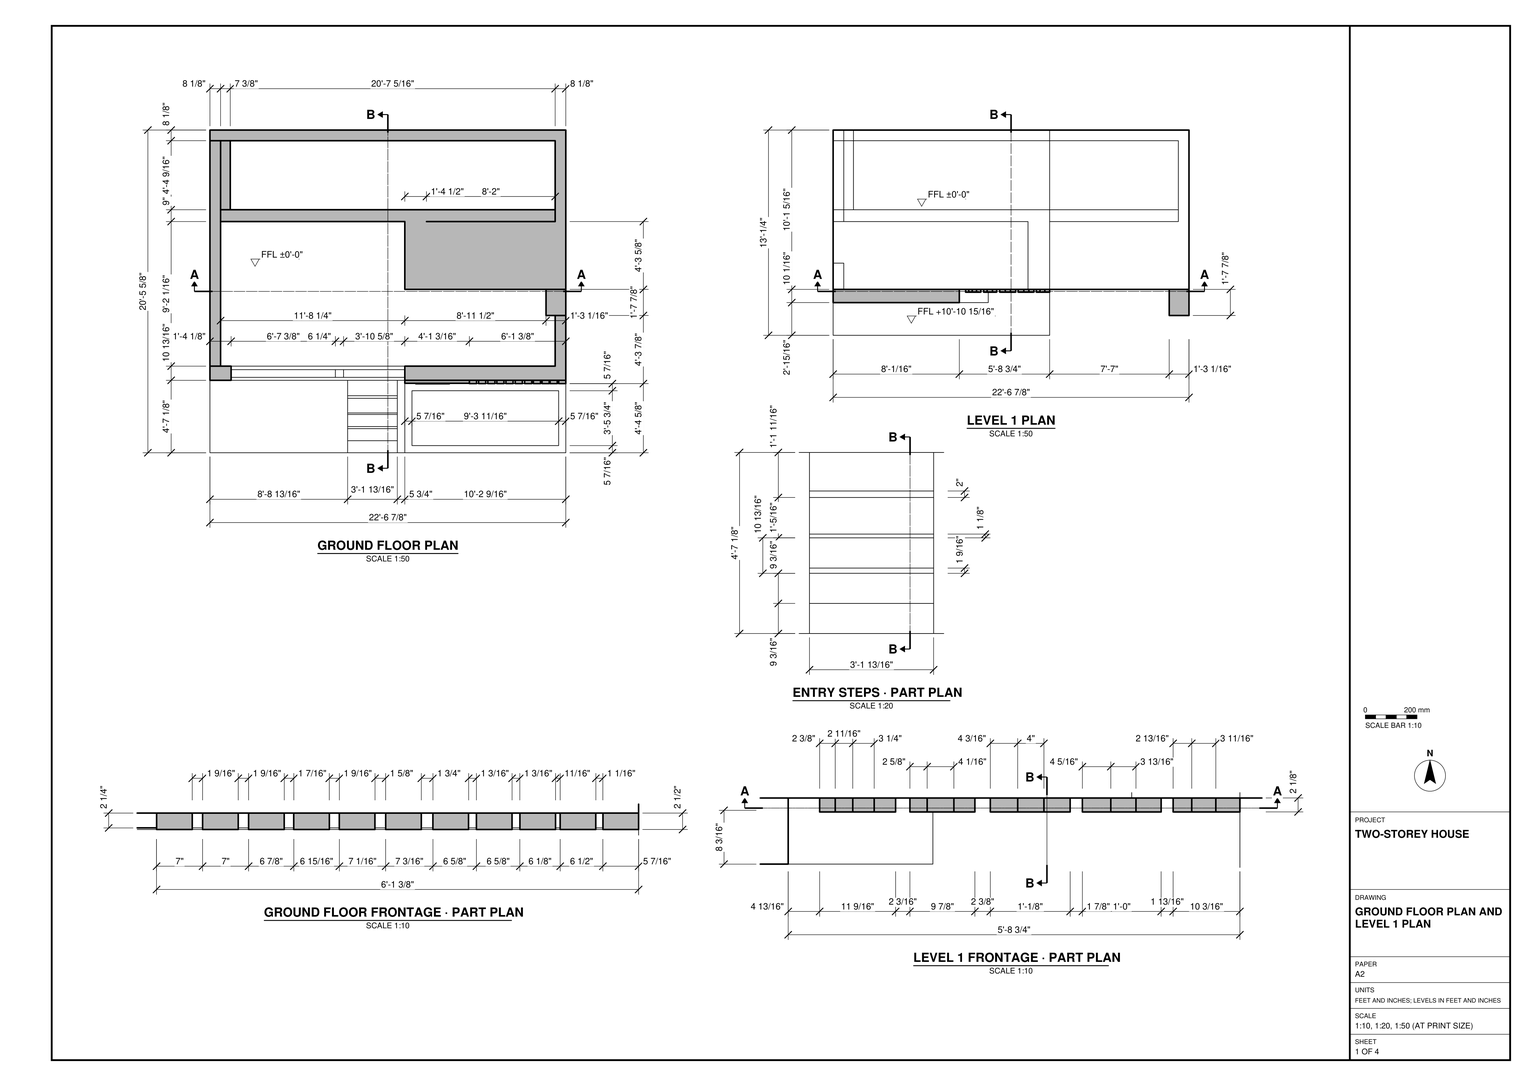
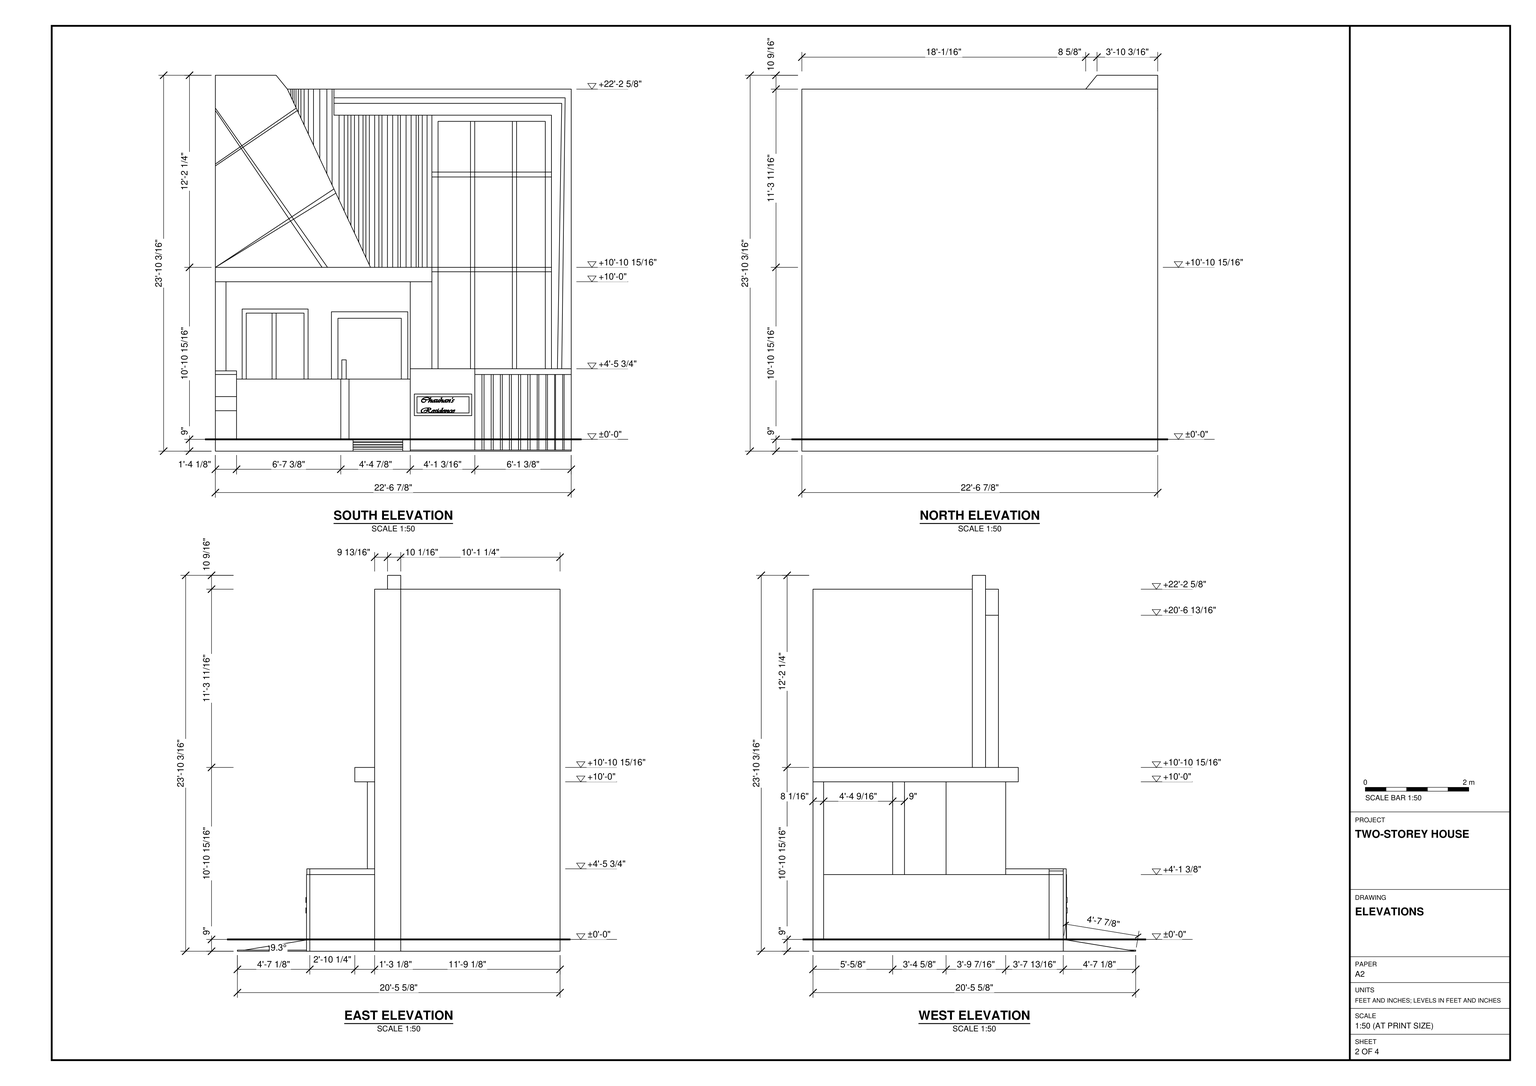
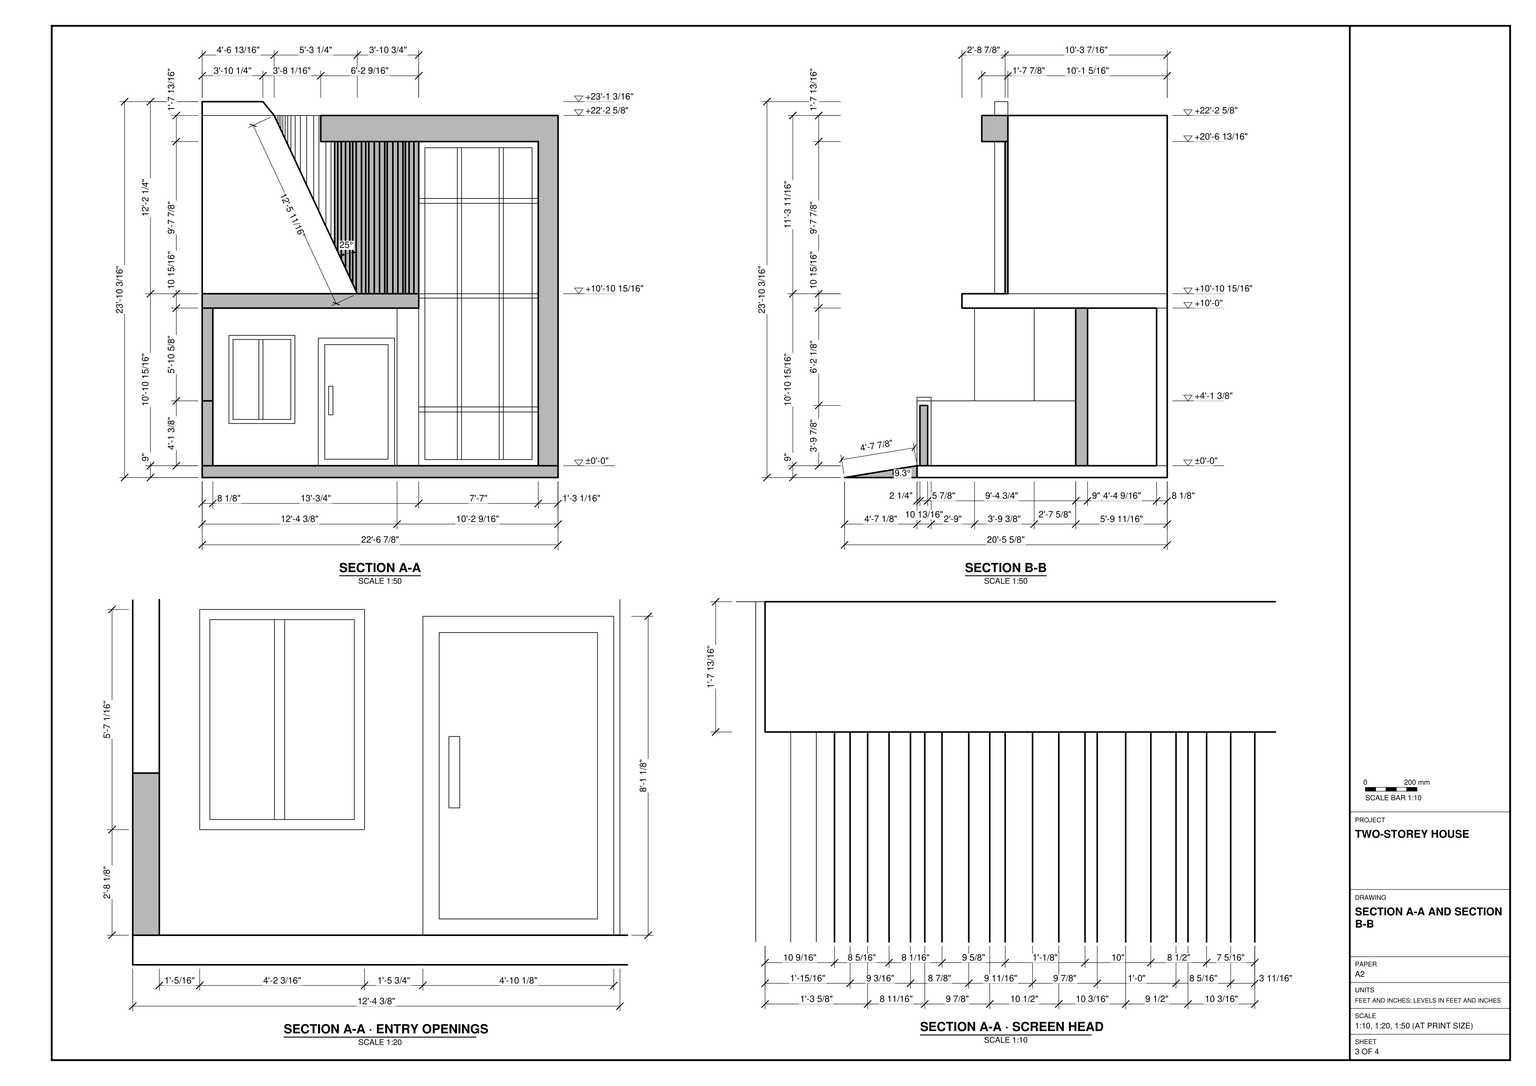
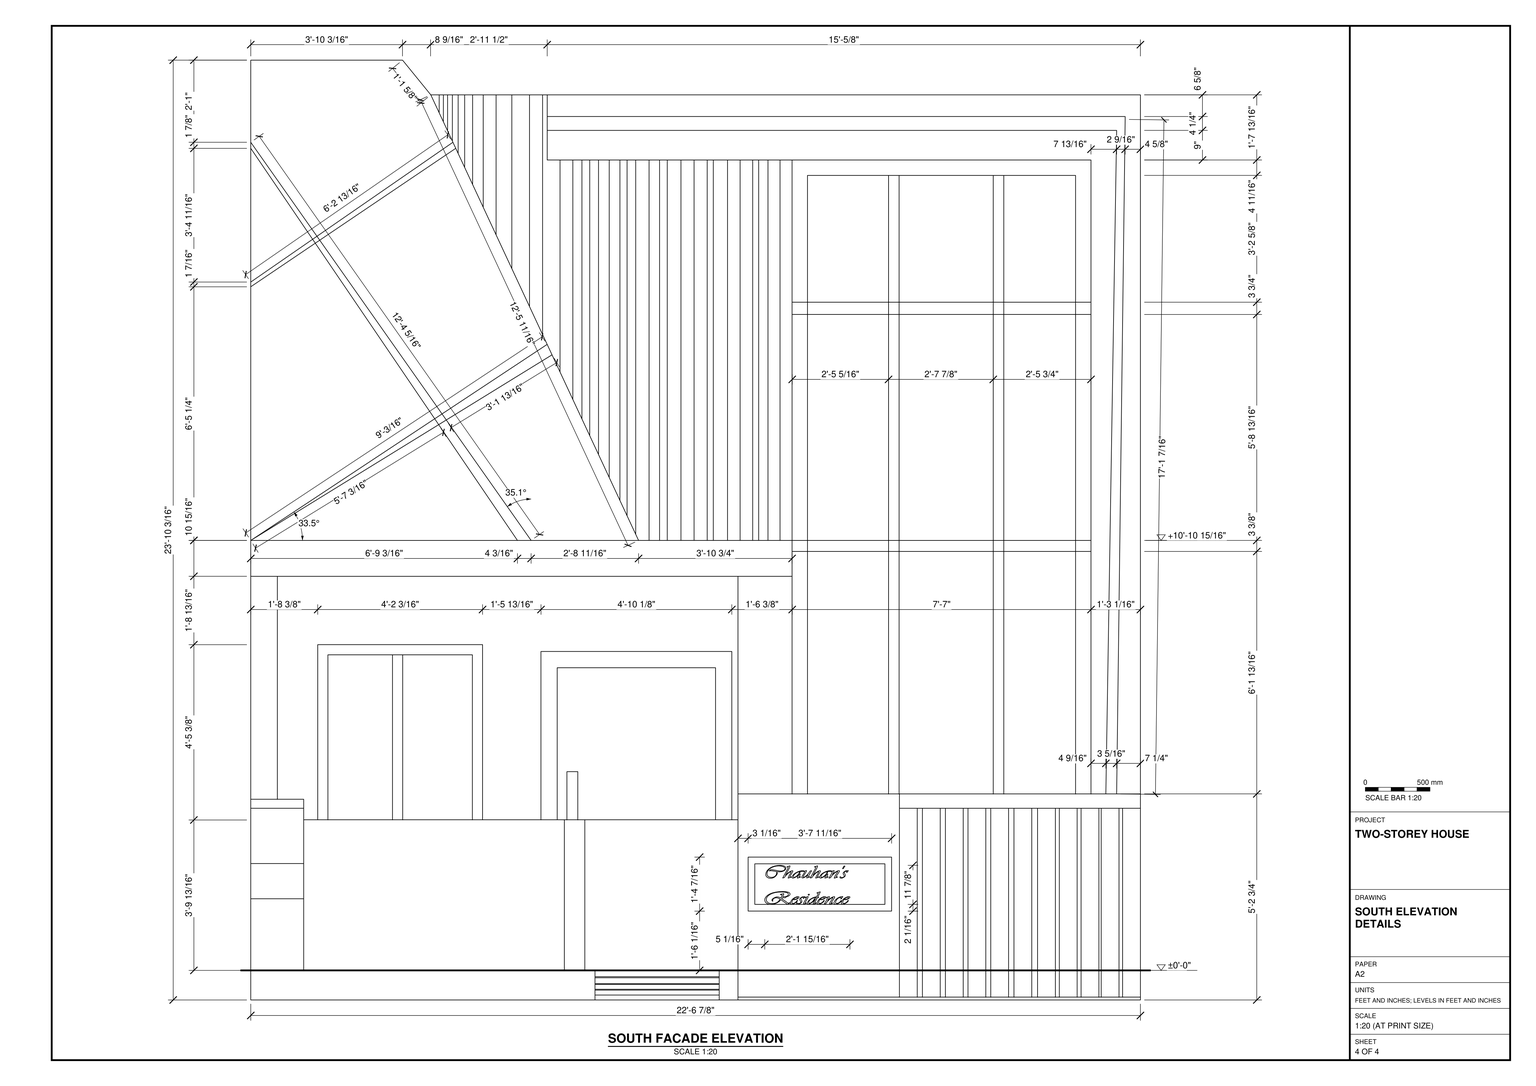
Build the two-storey house in SketchUp from task_files/diagram_01.pdf. Work in feet and inches. The overall dimensions are 22'-6 7/8" across the south frontage, 20'-5 5/8" from front to back and 23'-10 3/16" high. Set the ground floor at ±0'-0" and Level 1 at +10'-10 15/16".

Use the plans to set out the walls at their drawn thicknesses and the sections to locate the base slab, projecting Level 1 slab and roof edge. At the south entrance, model the steps, adjoining sloped approach and low frontage elements. Set the framed door and divided window back from the frontage, beneath the projecting slab. To their right, carry the tall glazed bay past Level 1 without interrupting it with the slab edge. Match its mullions, horizontal divisions and outer frame to section A-A. Above the entrance, fit the vertical screen between the glazed bay and the panel with the sloping edge. Follow the south elevation for the diagonal joints on that panel and the part plans for the spacing of the frontage members.

Keep walls, slabs and roof elements in separate groups or components. Group each furniture or joinery piece separately and use components for repeated parts. Any decor or loose items shown may be represented by suitable library components. Save one SketchUp model as output_files/two_storey_house_with_a_screened_south_frontage.skp.

# SketchUp Ruby script. Lengths in inches.
U = 1.inch
M = Sketchup.active_model
def pt(a) = Geom::Point3d.new(a.map { |v| v * U })
def face(e, loops, mat)
  f = e.add_face(loops[0].map { |a| pt(a) })
  loops[1..].each { |l| e.add_face(l.map { |a| pt(a) }).erase! }
  f.material = f.back_material = mat if mat
  f
end
# faces: each face lists its corners as indices into pts; further lists are holes
def faces(e, pts, list, mat = nil) = list.each { |f| face(e, (f[0].is_a?(Array) ? f : [f]).map { |l| l.map { |i| pts[i] } }, mat) }
# xy, xz, yz: faces in a plane at the given z, y or x. An outline is a flat list of corners, or four numbers for a rectangle; further outlines are holes
def ring(l) = l.size == 4 ? [[l[0], l[1]], [l[2], l[1]], [l[2], l[3]], [l[0], l[3]]] : l.each_slice(2).to_a
def flat(e, list, mat, &to3) = list.each { |f| face(e, (f[0].is_a?(Array) ? f : [f]).map { |l| ring(l).map { |u, v| to3.(u, v) } }, mat) }
def xy(e, z, list, mat = nil) = flat(e, list, mat) { |x, y| [x, y, z] }
def xz(e, y, list, mat = nil) = flat(e, list, mat) { |x, z| [x, y, z] }
def yz(e, x, list, mat = nil) = flat(e, list, mat) { |y, z| [x, y, z] }
def lines(e, pts, list) = list.each { |a, b| e.add_line(pt(pts[a]), pt(pts[b])) }
# prism: a flat outline (further loops are holes) pulled along v
def prism(e, loops, v, mat = nil)
  f = face(e, loops, mat); d = Geom::Vector3d.new(v.map { |x| x * U })
  f.pushpull(f.normal.samedirection?(d) ? d.length : -d.length)
end
def box(e, o, s, mat = nil) = prism(e, [[o, [o[0] + s[0], o[1], o[2]], [o[0] + s[0], o[1] + s[1], o[2]], [o[0], o[1] + s[1], o[2]]]], [0, 0, s[2]], mat)
def at(x, y, z, deg = 0) = Geom::Transformation.translation(pt([x, y, z])) * Geom::Transformation.rotation(ORIGIN, Z_AXIS, deg.degrees)
def axes(o, x, y, z) = Geom::Transformation.new([*x, 0, *y, 0, *z, 0, *pt(o).to_a, 1])
def part(name) = M.definitions.add(name)
# library, detail: a bought-in or finely detailed component or shape, given as its bounding box
def library(name, o, s) = part(name).tap { |d| box(d.entities, o, s) }
def detail(e, o, s) = box(e.add_group.entities, o, s)
def put(e, d, t, mat = nil) = e.add_instance(d, t).tap { |i| i.material = mat if mat }
def group(e, t, mat = nil) = e.add_group.tap { |g| g.transformation = t; g.material = mat if mat }.entities
root = M.entities
M.materials.add("[0014_DarkSalmon]").color = [242, 155, 126]
M.materials.add("[Asphalt New]").color = [67, 60, 62]
M.materials.add("[Blacktop New]").color = [81, 81, 81]
M.materials.add("[Concrete Aggregate Smoke]").color = [154, 150, 148]
M.materials.add("[Concrete Form 4x8]").color = [167, 170, 168]
M.materials.add("[Formica Beige]").color = [211, 187, 149]
M.materials.add("[Formica Graystone]").color = [149, 146, 135]
M.materials.add("[Formica Laminate Dark]").color = [50, 53, 60]
M.materials.add("[Formica Laminate Light]").color = [213, 189, 164]
M.materials.add("[Formica Speckled Grey]").color = [94, 105, 111]
M.materials.add("[Grass Dark Green]").color = [106, 157, 55]
M.materials.add("[Marble Carrara Floor Tile]").color = [204, 208, 219]
M.materials.add("[Marble Carrara Gold Floor Tile]").color = [225, 223, 217]
M.materials.add("[Polished Concrete New]").color = [200, 200, 203]
M.materials.add("[Polished Concrete Old]").color = [229, 229, 229]
M.materials.add("[Terrazzo Tile Accent]").color = [224, 221, 217]
M.materials.add("[Translucent Glass Safety]").color = [204, 235, 244]
M.materials["[Translucent Glass Safety]"].alpha = 0.5
M.materials.add("[Translucent Resin Crush Gray]").color = [184, 184, 184]
M.materials["[Translucent Resin Crush Gray]"].alpha = 0.8
M.materials.add("[Wood Cherry Original]").color = [119, 67, 33]
M.materials.add("[Wood Cherry Original]1").color = [152, 86, 42]
M.materials.add("[Wood Veneer 01]").color = [76, 44, 23]
c1 = library("Chauhan's Reside",[0.93,0,0],[38.14,23.39,12])
xy(root,0,[[0,0,148.36,55.13],[[148.36,0,270.9,52.63],[153.79,5.43,265.47,47.2]],[148.36,52.63,197.52,52.88],[197.52,52.63,202.95,52.88],[202.95,52.63,204.52,52.88],
  [204.52,52.63,209.95,52.88],[209.95,52.63,211.52,52.88],[211.52,52.63,216.95,52.88],[216.95,52.63,218.4,52.88],[218.4,52.63,223.82,52.88],
  [223.82,52.63,225.33,52.88],[225.33,52.63,230.76,52.88],[230.76,52.63,232.4,52.88],[232.4,52.63,237.82,52.88],[237.82,52.63,239.58,52.88],
  [239.58,52.63,245.01,52.88],[245.01,52.63,246.21,52.88],[246.21,52.63,251.63,52.88],[251.63,52.63,252.83,52.88],[252.83,52.63,258.26,52.88],
  [258.26,52.63,258.96,52.88],[258.96,52.63,264.38,52.88],[264.38,52.63,265.48,52.88],[265.48,52.63,270.9,52.88],[148.36,52.88,197.52,55.13],
  [197.52,52.88,202.95,55.13],[202.95,52.88,204.52,55.13],[204.52,52.88,209.95,55.13],[209.95,52.88,211.52,55.13],[211.52,52.88,216.95,55.13],
  [216.95,52.88,218.4,55.13],[218.4,52.88,223.82,55.13],[223.82,52.88,225.33,55.13],[225.33,52.88,230.76,55.13],[230.76,52.88,232.4,55.13],
  [232.4,52.88,237.82,55.13],[237.82,52.88,239.58,55.13],[239.58,52.88,245.01,55.13],[245.01,52.88,246.21,55.13],[246.21,52.88,251.63,55.13],
  [251.63,52.88,252.83,55.13],[252.83,52.88,258.26,55.13],[258.26,52.88,258.96,55.13],[258.96,52.88,264.38,55.13],[264.38,52.88,265.48,55.13],
  [265.48,52.88,270.9,55.13],[0,55.13,270.9,245.65]])
xy(root,0,[[153.79,5.43,265.47,47.2]],"[Grass Dark Green]")
xy(root,0.875,[[[148.36,0,270.9,52.63],[153.79,5.43,265.47,47.2]]],"[Translucent Resin Crush Gray]")
xy(root,9,[[16.12,55.13,148.36,57.38],[16.12,57.38,148.36,63.26],[16.12,63.26,148.36,65.92],[0,65.92,8.1,237.55],[255.85,104.48,262.81,124.36],
  [262.81,104.48,270.9,124.36],[148.36,124.36,164.83,175.99],[8.1,175.99,262.81,185],[8.1,185,15.48,237.55],[15.48,185,262.81,237.55]])
xy(root,9,[[8.1,65.92,262.81,65.92,262.81,104.48,255.85,104.48,255.85,124.36,148.36,124.36,148.36,175.99,8.1,175.99]],"[Marble Carrara Floor Tile]")
xy(root,54.875,[[95.49,57.38,101.72,63.26]],"[Formica Graystone]")
xy(root,54.875,[[16.12,57.38,95.49,63.26],[101.72,57.38,148.36,63.26]],"[Formica Laminate Dark]")
xy(root,58.375,[[0,55.13,16.12,65.92],[148.36,55.13,148.36,65.92,262.81,65.92,262.81,104.48,270.9,104.48,270.9,55.13],[0,98.95,8.1,144.35]])
xy(root,58.375,[[0,65.92,8.1,98.95],[0,144.35,8.1,237.55]],"[Formica Graystone]")
xy(root,58.375,[[197.52,52.63,202.95,55.13],[204.52,52.63,209.95,55.13],[211.52,52.63,216.95,55.13],[218.4,52.63,223.82,55.13],[225.33,52.63,230.76,55.13],
  [232.4,52.63,237.82,55.13],[239.58,52.63,245.01,55.13],[246.21,52.63,251.63,55.13],[252.83,52.63,258.26,55.13],[258.96,52.63,264.38,55.13],
  [265.48,52.63,270.9,55.13]],"[Wood Cherry Original]1")
xy(root,61.125,[[0,55.13,16.12,65.92]],"[Asphalt New]")
xy(root,62.75,[[148.36,52.88,197.52,55.13]])
xy(root,62.75,[[148.36,55.13,270.9,55.13,270.9,104.48,262.81,104.48,262.81,65.92,148.36,65.92]],"[Asphalt New]")
xy(root,129,[[0,89.38,8.1,98.95],[0,98.95,8.1,144.35],[148.36,124.36,164.83,124.36,164.83,185,8.1,185,8.1,175.99,148.36,175.99],[0,175.99,8.1,185],[164.83,175.99,262.81,185],
  [0,185,8.1,237.55],[8.1,185,15.48,237.55],[15.48,185,164.83,237.55],[164.83,185,262.81,237.55]])
xy(root,129,[[8.1,89.38,8.1,144.35,0,144.35,0,175.99,148.36,175.99,148.36,124.36,164.83,124.36,164.83,89.38]],"[0014_DarkSalmon]")
xy(root,139.9375,[[0,114.3,118.09,124.36],[118.09,122.23,121.28,124.36],[121.28,122.23,124.48,124.36],[126.83,122.23,131,124.36],[131,122.23,134.99,124.36],
  [134.99,122.23,138.99,124.36],[140.85,122.23,145.17,124.36],[145.17,122.23,149.01,124.36],[149.01,122.23,152.84,124.36],[154.66,122.23,157.5,124.36],
  [157.5,122.23,161.17,124.36],[161.17,122.23,164.83,124.36]])
xy(root,139.9375,[[0,89.38,164.83,89.38,164.83,122.23,154.66,122.23,154.66,124.36,152.84,124.36,152.84,122.23,140.85,122.23,140.85,124.36,138.99,124.36,138.99,122.23,126.83,122.23,126.83,124.36,124.48,124.36,124.48,122.23,118.09,122.23,118.09,114.3,0,114.3]],"[Formica Speckled Grey]")
xy(root,255.79,[[100.85,122.23,103.22,124.36],[103.22,122.23,105.89,124.36],[105.89,122.23,109.15,124.36],[109.15,122.23,112.41,124.36],[114.59,122.23,117.22,124.36],
  [117.22,122.23,121.28,124.36],[121.28,122.23,124.48,124.36],[126.83,122.23,131,124.36],[131,122.23,134.99,124.36],[134.99,122.23,138.99,124.36],
  [140.85,122.23,145.17,124.36],[145.17,122.23,149.01,124.36],[149.01,122.23,152.84,124.36],[154.66,122.23,157.5,124.36],[157.5,122.23,161.17,124.36],
  [161.17,122.23,164.83,124.36]])
xy(root,255.79,[[90.27,104.48,90.27,124.36,100.85,124.36,100.85,122.23,112.41,122.23,112.41,124.36,114.59,124.36,114.59,122.23,124.48,122.23,124.48,124.36,126.83,124.36,126.83,122.23,138.99,122.23,138.99,124.36,140.85,124.36,140.85,122.23,152.84,122.23,152.84,124.36,154.66,124.36,154.66,122.23,164.83,122.23,164.83,124.36,255.85,124.36,255.85,104.48]],"[Formica Laminate Dark]")
xy(root,275.625,[[90.27,104.48,270.9,124.36]],"[Formica Laminate Dark]")
xy(root,275.625,[[0,124.36,270.9,245.65]],"[Terrazzo Tile Accent]")
xy(root,286.1875,[[0,114.3,46.23,124.36]],"[Blacktop New]")
xz(root,0,[[148.36,0,270.9,0.875]],"[Translucent Resin Crush Gray]")
xz(root,5.43,[[153.79,0,265.47,0.875]])
xz(root,47.2,[[153.79,0,197.52,0.875],[197.52,0,202.95,0.875],[202.95,0,204.52,0.875],[204.52,0,209.95,0.875],[209.95,0,211.52,0.875],
  [211.52,0,216.95,0.875],[216.95,0,218.4,0.875],[218.4,0,223.82,0.875],[223.82,0,225.33,0.875],[225.33,0,230.76,0.875],
  [230.76,0,232.4,0.875],[232.4,0,237.82,0.875],[237.82,0,239.58,0.875],[239.58,0,245.01,0.875],[245.01,0,246.21,0.875],
  [246.21,0,251.63,0.875],[251.63,0,252.83,0.875],[252.83,0,258.26,0.875],[258.26,0,258.96,0.875],[258.96,0,264.38,0.875],
  [264.38,0,265.47,0.875]])
xz(root,52.63,[[148.36,0,197.52,0.875],[197.52,0,202.95,0.875],[202.95,0,204.52,0.875],[204.52,0,209.95,0.875],[209.95,0,211.52,0.875],
  [211.52,0,216.95,0.875],[216.95,0,218.4,0.875],[218.4,0,223.82,0.875],[223.82,0,225.33,0.875],[225.33,0,230.76,0.875],
  [230.76,0,232.4,0.875],[232.4,0,237.82,0.875],[237.82,0,239.58,0.875],[239.58,0,245.01,0.875],[245.01,0,246.21,0.875],
  [246.21,0,251.63,0.875],[251.63,0,252.83,0.875],[252.83,0,258.26,0.875],[258.26,0,258.96,0.875],[258.96,0,264.38,0.875],
  [264.38,0,265.48,0.875],[265.48,0,270.9,0.875]])
xz(root,52.63,[[197.52,0.875,202.95,58.375],[204.52,0.875,209.95,58.375],[211.52,0.875,216.95,58.375],[218.4,0.875,223.82,58.375],[225.33,0.875,230.76,58.375],
  [232.4,0.875,237.82,58.375],[239.58,0.875,245.01,58.375],[246.21,0.875,251.63,58.375],[252.83,0.875,258.26,58.375],[258.96,0.875,264.38,58.375],
  [265.48,0.875,270.9,58.375]],"[Wood Cherry Original]1")
xz(root,52.88,[[[151.45,27.0625,195.14,43.5],[153.49,29.1,193.1,41.46]]],"[Formica Beige]")
xz(root,52.88,[[153.49,29.1,193.1,41.46]],"[Formica Speckled Grey]")
xz(root,52.88,[[[148.36,0,197.52,62.75],[151.45,27.0625,195.14,43.5]]],"[Polished Concrete New]")
xz(root,55.13,[[16.12,0,148.36,9],[148.36,0,197.52,58.375],[197.52,0,202.95,58.375],[204.52,0,209.95,58.375],[211.52,0,216.95,58.375],
  [218.4,0,223.82,58.375],[225.33,0,230.76,58.375],[232.4,0,237.82,58.375],[239.58,0,245.01,58.375],[246.21,0,251.63,58.375],
  [252.83,0,258.26,58.375],[258.96,0,264.38,58.375],[265.48,0,270.9,58.375],[148.36,58.375,197.52,62.75]])
xz(root,55.13,[[0,30.82,16.12,41.54],[0,58.375,16.12,61.125]],"[Asphalt New]")
xz(root,55.13,[[202.95,0,204.52,58.375],[209.95,0,211.52,58.375],[216.95,0,218.4,58.375],[223.82,0,225.33,58.375],[230.76,0,232.4,58.375],
  [237.82,0,239.58,58.375],[245.01,0,246.21,58.375],[251.63,0,252.83,58.375],[258.26,0,258.96,58.375],[264.38,0,265.48,58.375]],"[Formica Beige]")
xz(root,55.13,[[0,0,16.12,30.82],[0,41.54,16.12,58.375]],"[Formica Graystone]")
xz(root,55.13,[[197.52,58.375,270.9,62.75]],"[Formica Laminate Dark]")
xz(root,57.38,[[95.49,9,101.72,54.875]],"[Concrete Aggregate Smoke]")
xz(root,57.38,[[16.12,9,95.49,54.875],[101.72,9,148.36,54.875]],"[Formica Laminate Dark]")
xz(root,63.26,[[16.12,9,148.36,54.875]],"[Formica Laminate Dark]")
xz(root,65.92,[[0,9,8.1,58.375],[259.91,9,262.81,58.375]])
xz(root,65.92,[[0,58.375,8.1,61.125],[8.1,58.375,16.12,61.125],[148.36,58.375,259.91,62.75],[259.91,58.375,262.81,62.75]],"[Asphalt New]")
xz(root,65.92,[[8.1,9,16.12,58.375],[148.36,9,259.91,58.375]],"[Formica Graystone]")
xz(root,89.38,[[0,129,164.83,139.9375]],"[Formica Graystone]")
xz(root,98.95,[[0,58.375,8.1,129]],"[Formica Graystone]")
xz(root,104.48,[[262.81,9,270.9,58.375],[262.81,58.375,270.9,62.75]])
xz(root,104.48,[[260.375,62.75,263.66,62.75,266.25,268.15,266.25,269.03,90.27,269.03,90.27,264.8,263.66,264.8]],"[Formica Beige]")
xz(root,104.48,[[255.85,9,262.81,9,262.81,62.75,260.375,62.75,263.66,264.8,90.27,264.8,90.27,255.79,255.85,255.79],[263.66,62.75,270.9,62.75,270.9,275.625,90.27,275.625,90.27,269.03,266.25,269.03,266.25,268.15]],"[Formica Laminate Dark]")
xz(root,114.3,[[0,139.9375,56.01,176.99,19.65,230.45,0,217.18],[0,139.9375,81.21,139.9375,57.23,175.2],[85.37,139.9375,118.09,139.9375,91.74,196.46,59.54,176.62],[58.24,178.46,90.25,199.64,62.42,259.34,21,231.36],[0,218.62,18.83,231.65,0,259.34],
  [20.16,232.56,61.56,261.18,54.82,275.625,46.23,286.1875,0,286.1875,0,261.18]],"[Blacktop New]")
xz(root,114.3,[[0,139.9375,57.23,175.2,56.01,176.99],[81.21,139.9375,85.37,139.9375,59.54,176.62,57.23,175.2],[57.23,175.2,59.54,176.62,58.24,178.46,56.01,176.99],[59.54,176.62,91.74,196.46,90.25,199.64,58.24,178.46],[56.01,176.99,58.24,178.46,21,231.36,19.65,230.45],
  [0,217.18,19.65,230.45,18.83,231.65,0,218.62],[19.65,230.45,21,231.36,20.16,232.56,18.83,231.65],[21,231.36,62.42,259.34,61.56,261.18,20.16,232.56],[18.83,231.65,20.16,232.56,0,261.18,0,259.34]],"[Polished Concrete Old]")
xz(root,122.23,[[118.09,139.9375,121.28,139.9375,121.28,255.79,117.22,255.79,117.22,141.8],[121.28,139.9375,124.48,255.79],[126.83,139.9375,131,255.79],[131,139.9375,134.99,255.79],[134.99,139.9375,138.99,255.79],
  [140.85,139.9375,145.17,255.79],[145.17,139.9375,149.01,255.79],[149.01,139.9375,152.84,255.79],[154.66,139.9375,157.5,255.79],[157.5,139.9375,161.17,255.79],
  [161.17,139.9375,164.83,255.79],[117.22,141.8,117.22,255.79,114.59,255.79,114.59,147.4375],[112.41,152.11,112.41,255.79,109.15,255.79,109.15,159.1],[109.15,159.1,109.15,255.79,105.89,255.79,105.89,166.1],[105.89,166.1,105.89,255.79,103.22,255.79,103.22,171.83],
  [103.22,171.83,103.22,255.79,100.85,255.79,100.85,176.92]],"[Wood Cherry Original]1")
xz(root,124.36,[[255.85,9,255.85,255.79,90.27,255.79,90.27,275.625,270.9,275.625,270.9,9],[0,139.9375,0,275.625,54.82,275.625,57.38,270.15,58.65,267.41,59.93,264.67,61.39,261.54,63.15,257.76,65.13,253.51,67.5625,248.3,70.78,241.4,74.7,232.99,79.5,222.7,84.88,211.15,88.86,202.63,94.17,191.22,98.08,182.85,100.85,176.92,103.22,171.83,105.89,166.1,109.15,159.1,112.41,152.11,114.59,147.4375,117.22,141.8,118.09,139.9375],[118.09,139.9375,117.22,141.8,117.22,255.79,121.28,255.79,121.28,139.9375],[121.28,139.9375,124.48,255.79],[126.83,139.9375,131,255.79],
  [131,139.9375,134.99,255.79],[134.99,139.9375,138.99,255.79],[140.85,139.9375,145.17,255.79],[145.17,139.9375,149.01,255.79],[149.01,139.9375,152.84,255.79],
  [154.66,139.9375,157.5,255.79],[157.5,139.9375,161.17,255.79],[161.17,139.9375,164.83,255.79],[117.22,141.8,114.59,147.4375,114.59,255.79,117.22,255.79],[112.41,152.11,109.15,159.1,109.15,255.79,112.41,255.79],
  [109.15,159.1,105.89,166.1,105.89,255.79,109.15,255.79],[105.89,166.1,103.22,171.83,103.22,255.79,105.89,255.79],[103.22,171.83,100.85,176.92,100.85,255.79,103.22,255.79]])
xz(root,124.36,[[0,275.625,0,286.1875,46.23,286.1875,54.82,275.625]],"[Asphalt New]")
xz(root,124.36,[[124.48,139.9375,126.83,255.79],[138.99,139.9375,140.85,255.79],[152.84,139.9375,154.66,255.79],[114.59,147.4375,114.59,255.79,112.41,255.79,112.41,152.11],[100.85,176.92,100.85,255.79,98.08,255.79,98.08,182.85]],"[Formica Beige]")
xz(root,124.36,[[148.36,9,164.83,129]],"[Polished Concrete New]")
xz(root,124.36,[[169.53,13.69,194.21,49.93],[197.42,13.69,226.09,49.93],[229.3,13.69,251.16,49.93],[169.53,53.76,194.21,136.58],[197.42,53.76,226.09,136.58],
  [229.3,53.76,251.16,136.58],[169.53,139.9375,194.21,208.76],[197.42,139.9375,226.09,208.76],[229.3,139.9375,251.16,208.76],[169.53,212.48,194.21,251.09],
  [197.42,212.48,226.09,251.09],[229.3,212.48,251.16,251.09]],"[Translucent Glass Safety]")
xz(root,124.36,[[98.08,182.85,98.08,255.79,94.17,255.79,94.17,191.22]],"[Wood Cherry Original]")
xz(root,124.36,[[94.17,191.22,94.17,255.79,90.27,255.79,90.27,275.625,88.86,275.625,88.86,202.63],[88.86,202.63,88.86,275.625,84.88,275.625,84.88,211.15],[84.88,211.15,84.88,275.625,79.5,275.625,79.5,222.7],[79.5,222.7,79.5,275.625,74.7,275.625,74.7,232.99],[74.7,232.99,74.7,275.625,70.78,275.625,70.78,241.4],
  [70.78,241.4,70.78,275.625,67.5625,275.625,67.5625,248.3],[67.5625,248.3,67.5625,275.625,65.13,275.625,65.13,253.51],[65.13,253.51,65.13,275.625,63.15,275.625,63.15,257.76],[63.15,257.76,63.15,275.625,61.39,275.625,61.39,261.54],[61.39,261.54,61.39,275.625,59.93,275.625,59.93,264.67],
  [59.93,264.67,59.93,275.625,58.65,275.625,58.65,267.41],[58.65,267.41,58.65,275.625,57.38,275.625,57.38,270.15],[57.38,270.15,57.38,275.625,54.82,275.625]],"[Wood Cherry Original]1")
xz(root,124.36,[[164.83,9,255.85,9,255.85,49.93,251.16,49.93,251.16,13.69,169.53,13.69,169.53,49.93,164.83,49.93],[194.21,13.69,197.42,49.93],[226.09,13.69,229.3,49.93],[164.83,49.93,169.53,53.76],[169.53,49.93,194.21,53.76],
  [194.21,49.93,197.42,53.76],[197.42,49.93,226.09,53.76],[226.09,49.93,229.3,53.76],[229.3,49.93,251.16,53.76],[251.16,49.93,255.85,53.76],
  [164.83,53.76,169.53,136.58],[194.21,53.76,197.42,136.58],[226.09,53.76,229.3,136.58],[251.16,53.76,255.85,136.58],[164.83,136.58,169.53,139.9375],
  [169.53,136.58,194.21,139.9375],[194.21,136.58,197.42,139.9375],[197.42,136.58,226.09,139.9375],[226.09,136.58,229.3,139.9375],[229.3,136.58,251.16,139.9375],
  [251.16,136.58,255.85,139.9375],[164.83,139.9375,169.53,208.76],[194.21,139.9375,197.42,208.76],[226.09,139.9375,229.3,208.76],[251.16,139.9375,255.85,208.76],
  [164.83,208.76,169.53,212.48],[169.53,208.76,194.21,212.48],[194.21,208.76,197.42,212.48],[197.42,208.76,226.09,212.48],[226.09,208.76,229.3,212.48],
  [229.3,208.76,251.16,212.48],[251.16,208.76,255.85,212.48],[164.83,212.48,169.53,212.48,169.53,251.09,251.16,251.09,251.16,212.48,255.85,212.48,255.85,255.79,164.83,255.79],[194.21,212.48,197.42,251.09],[226.09,212.48,229.3,251.09]],"[Wood Veneer 01]")
xz(root,144.35,[[0,58.375,8.1,129]],"[Formica Graystone]")
xz(root,175.99,[[164.83,9,262.81,129]])
xz(root,175.99,[[[8.1,9,88.36,9,88.36,106.125,146.48,106.125,146.48,9,148.36,9,148.36,129,8.1,129],[20.39,41.14,70.58,108.2]]],"[0014_DarkSalmon]")
xz(root,175.99,[[96.27,47.78,99.58,69.53]],"[Formica Laminate Light]")
xz(root,175.99,[[23.49,44.24,43.16,105.11],[46.26,44.24,67.49,105.11]],"[Translucent Glass Safety]")
xz(root,175.99,[[[20.39,41.14,70.58,108.2],[23.49,44.24,67.49,105.11]],[43.16,44.24,46.26,105.11]],"[Wood Cherry Original]")
xz(root,175.99,[[[88.36,9,146.48,106.125],[93.3125,13.95,141.53,101.17]],[[93.3125,13.95,141.53,101.17],[96.27,47.78,99.58,69.53]]],"[Wood Veneer 01]")
xz(root,185,[[8.1,9,15.48,129],[15.48,9,262.81,129]])
xz(root,237.55,[[0,9,8.1,58.375],[8.1,9,15.48,129],[15.48,9,262.81,129]])
xz(root,237.55,[[0,58.375,8.1,129]],"[Formica Graystone]")
xz(root,245.65,[[0,0,270.9,9],[0,9,270.9,275.625]],"[Terrazzo Tile Accent]")
yz(root,0,[[55.13,58.375,65.92,61.125]],"[Asphalt New]")
yz(root,0,[[114.3,139.9375,124.36,286.1875]],"[Blacktop New]")
yz(root,0,[[55.13,0,55.13,58.375,65.92,58.375,65.92,9,245.65,9,245.65,0],[65.92,9,237.55,58.375],[237.55,9,245.65,129],[98.95,58.375,144.35,129],[89.38,129,245.65,139.9375]],"[Formica Graystone]")
yz(root,0,[[124.36,139.9375,245.65,275.625]],"[Terrazzo Tile Accent]")
yz(root,8.1,[[175.99,9,185,58.375],[185,9,237.55,58.375]])
yz(root,8.1,[[65.92,9,175.99,58.375],[98.95,58.375,144.35,129]],"[0014_DarkSalmon]")
yz(root,8.1,[[175.99,58.375,185,129],[185,58.375,237.55,129]],"[Formica Beige]")
yz(root,15.48,[[185,9,237.55,129]])
yz(root,16.12,[[57.38,9,63.26,54.875]])
yz(root,16.12,[[55.13,58.375,65.92,61.125]],"[Asphalt New]")
yz(root,16.12,[[55.13,9,57.38,9,57.38,54.875,63.26,54.875,63.26,9,65.92,9,65.92,58.375,55.13,58.375]],"[Concrete Form 4x8]")
yz(root,90.27,[[104.48,255.79,124.36,275.625]],"[Formica Laminate Dark]")
yz(root,100.85,[[122.23,176.92,124.36,178.91]])
yz(root,100.85,[[122.23,178.91,124.36,255.79]],"[Wood Cherry Original]1")
yz(root,103.22,[[122.23,171.83,124.36,255.79]])
yz(root,105.89,[[122.23,166.1,124.36,255.79]])
yz(root,109.15,[[122.23,159.1,124.36,249.85],[122.23,249.85,124.36,255.79]])
yz(root,112.41,[[122.23,152.11,124.36,255.79]],"[Wood Cherry Original]1")
yz(root,114.59,[[122.23,147.4375,124.36,255.79]],"[Wood Cherry Original]1")
yz(root,117.22,[[122.23,141.8,124.36,255.79]])
yz(root,121.28,[[122.23,139.9375,124.36,255.79]])
yz(root,124.48,[[122.23,139.9375,124.36,255.79]],"[Wood Cherry Original]1")
yz(root,126.83,[[122.23,139.9375,124.36,255.79]],"[Wood Cherry Original]1")
yz(root,131,[[122.23,139.9375,124.36,255.79]])
yz(root,134.99,[[122.23,139.9375,124.36,255.79]])
yz(root,138.99,[[122.23,139.9375,124.36,255.79]],"[Wood Cherry Original]1")
yz(root,140.85,[[122.23,139.9375,124.36,255.79]],"[Wood Cherry Original]1")
yz(root,145.17,[[122.23,139.9375,124.36,255.79]])
yz(root,148.36,[[0,0,52.63,0.875],[52.88,0,55.13,9]])
yz(root,148.36,[[124.36,9,175.99,129]],"[0014_DarkSalmon]")
yz(root,148.36,[[55.13,58.375,65.92,62.75]],"[Asphalt New]")
yz(root,148.36,[[52.88,9,55.13,62.75],[55.13,9,55.13,58.375,65.92,58.375,65.92,9,63.26,9,63.26,54.875,57.38,54.875,57.38,9]],"[Concrete Form 4x8]")
yz(root,149.01,[[122.23,139.9375,124.36,255.79]])
yz(root,152.84,[[122.23,139.9375,124.36,255.79]],"[Wood Cherry Original]1")
yz(root,153.79,[[5.43,0,47.2,0.875]])
yz(root,154.66,[[122.23,139.9375,124.36,255.79]],"[Wood Cherry Original]1")
yz(root,157.5,[[122.23,139.9375,124.36,255.79]])
yz(root,161.17,[[122.23,139.9375,124.36,255.79]])
yz(root,164.83,[[124.36,129,175.99,139.9375],[175.99,129,185,139.9375],[185,129,237.55,139.9375]])
yz(root,164.83,[[89.38,129,124.36,139.9375]],"[Formica Graystone]")
yz(root,164.83,[[122.23,139.9375,124.36,208.76],[122.23,208.76,124.36,212.48],[122.23,212.48,124.36,255.79]],"[Wood Cherry Original]1")
yz(root,197.52,[[52.88,0,55.13,58.375],[52.88,58.375,55.13,62.75]])
yz(root,197.52,[[52.63,0,52.88,58.375]],"[Wood Cherry Original]1")
yz(root,202.95,[[52.63,0,55.13,58.375]],"[Wood Cherry Original]1")
yz(root,204.52,[[52.63,0,55.13,58.375]],"[Wood Cherry Original]1")
yz(root,209.95,[[52.63,0,55.13,58.375]],"[Wood Cherry Original]1")
yz(root,211.52,[[52.63,0,55.13,58.375]],"[Wood Cherry Original]1")
yz(root,216.95,[[52.63,0,55.13,58.375]],"[Wood Cherry Original]1")
yz(root,218.4,[[52.63,0,55.13,58.375]],"[Wood Cherry Original]1")
yz(root,223.82,[[52.63,0,55.13,58.375]],"[Wood Cherry Original]1")
yz(root,225.33,[[52.63,0,55.13,58.375]],"[Wood Cherry Original]1")
yz(root,230.76,[[52.63,0,55.13,58.375]],"[Wood Cherry Original]1")
yz(root,232.4,[[52.63,0,55.13,58.375]],"[Wood Cherry Original]1")
yz(root,237.82,[[52.63,0,55.13,58.375]],"[Wood Cherry Original]1")
yz(root,239.58,[[52.63,0,55.13,58.375]],"[Wood Cherry Original]1")
yz(root,245.01,[[52.63,0,55.13,58.375]],"[Wood Cherry Original]1")
yz(root,246.21,[[52.63,0,55.13,58.375]],"[Wood Cherry Original]1")
yz(root,251.63,[[52.63,0,55.13,58.375]],"[Wood Cherry Original]1")
yz(root,252.83,[[52.63,0,55.13,58.375]],"[Wood Cherry Original]1")
yz(root,255.85,[[104.48,9,124.36,255.79]],"[Formica Laminate Dark]")
yz(root,258.26,[[52.63,0,55.13,58.375]],"[Wood Cherry Original]1")
yz(root,258.96,[[52.63,0,55.13,58.375]],"[Wood Cherry Original]1")
yz(root,262.81,[[175.99,9,185,129],[185,9,237.55,129]])
yz(root,262.81,[[65.92,58.375,104.48,62.75]],"[Asphalt New]")
yz(root,262.81,[[65.92,9,104.48,58.375]],"[Formica Graystone]")
yz(root,264.38,[[52.63,0,55.13,58.375]],"[Wood Cherry Original]1")
yz(root,265.47,[[5.43,0,47.2,0.875]])
yz(root,265.48,[[52.63,0,55.13,58.375]],"[Wood Cherry Original]1")
yz(root,270.9,[[0,0,52.63,0.875]])
yz(root,270.9,[[55.13,0,104.48,58.375]],"[Formica Graystone]")
yz(root,270.9,[[104.48,0,124.36,9],[104.48,9,124.36,275.625],[55.13,58.375,104.48,62.75]],"[Formica Laminate Dark]")
yz(root,270.9,[[124.36,0,245.65,275.625]],"[Terrazzo Tile Accent]")
yz(root,270.9,[[52.63,0,55.13,58.375]],"[Wood Cherry Original]1")
p = [[57.38,124.36,270.15],[54.82,124.36,275.625],[54.82,114.3,275.625],[61.56,114.3,261.18],[62.42,114.3,259.34],[90.25,114.3,199.64],
  [91.74,114.3,196.46],[118.09,114.3,139.9375],[118.09,122.23,139.9375],[117.22,122.23,141.8],[114.59,122.23,147.4375],[114.59,124.36,147.4375],
  [112.41,124.36,152.11],[112.41,122.23,152.11],[109.15,122.23,159.1],[105.89,122.23,166.1],[103.22,122.23,171.83],[100.85,122.23,176.92],
  [100.85,124.36,176.92],[98.08,124.36,182.85],[94.17,124.36,191.22],[88.86,124.36,202.63],[84.88,124.36,211.15],[79.5,124.36,222.7],
  [74.7,124.36,232.99],[70.78,124.36,241.4],[67.5625,124.36,248.3],[65.13,124.36,253.51],[63.15,124.36,257.76],[61.39,124.36,261.54],
  [59.93,124.36,264.67],[58.65,124.36,267.41],[118.09,124.36,139.9375],[117.22,124.36,141.8],[109.15,124.36,159.1],[105.89,124.36,166.1],
  [103.22,124.36,171.83],[46.23,114.3,286.1875],[46.23,124.36,286.1875],[15.48,237.55,129],[15.48,245.65,129],[164.83,237.55,129],
  [164.83,245.65,129],[8.1,237.55,129],[8.1,245.65,129],[164.83,237.55,139.9375],[164.83,245.65,139.9375],[262.81,175.99,129],
  [262.81,175.99,237],[262.81,237.55,129],[262.81,237.55,237],[262.81,185,129],[262.81,185,237],[164.83,175.99,139.9375],
  [164.83,175.99,275.625],[164.83,185,139.9375],[164.83,185,275.625],[164.83,237.55,275.625],[104.82,43.4,7.08],[142.64,43.4,7.08],
  [104.82,30.28,4.94],[142.64,30.28,4.94],[104.82,19.93,3.25],[142.64,19.93,3.25]]
faces(root,p,[[0,1,2,3,4,5,6,7,8,9,10,11,12,13,14,15,16,17,18,19,20,21,22,23,24,25,26,27,28,29,30,31],[37,2,1,38]],"[Blacktop New]")
faces(root,p,[[32,33,9,8],[33,11,10,9],[12,34,14,13],[34,35,15,14],[35,36,16,15],[36,18,17,16]])
lines(root,p,[[39,40],[41,42],[43,44],[45,46],[47,48],[49,50],[51,52],[53,54],[55,56],[45,57],[58,59],[60,61],
  [62,63]])
put(root,c1,axes([155.89,52.88,29.1],[0.68,0,0],[0,0,0.50816],[0,-0.06,0]))
g1 = group(root,at(0,0,0),"[Marble Carrara Gold Floor Tile]")
xy(g1,0,[[0,0,148.36,52.88],[0,52.88,148.36,55.13]])
xz(g1,55.13,[[0,0,148.36,9]])
yz(g1,0,[[0,0,55.13,9,55.13,0]])
yz(g1,148.36,[[0,0,55.13,0,55.13,9]])
p = [[0,0,0],[104.82,0,0],[104.82,9.17,1.5],[104.82,18.34,2.99],[104.82,29.13,4.76],[104.82,41.42,6.76],
  [104.82,55.13,9],[0,55.13,9],[142.64,0,0],[142.64,9.17,1.5],[148.36,55.13,9],[142.64,55.13,9],
  [142.64,41.42,6.76],[142.64,29.13,4.76],[142.64,18.34,2.99],[148.36,0,0]]
faces(g1,p,[[0,1,2,3,4,5,6,7],[8,9,2,1],[10,11,12,13,14,9,8,15],[3,2,9,14],[4,3,14,13],[5,4,13,12],[6,5,12,11]])
